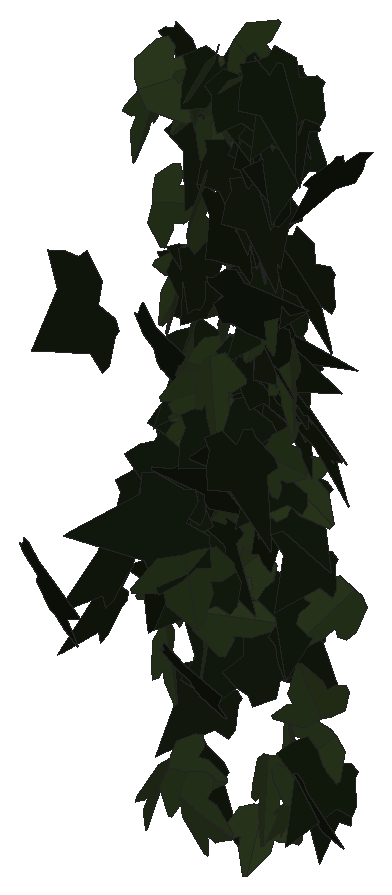
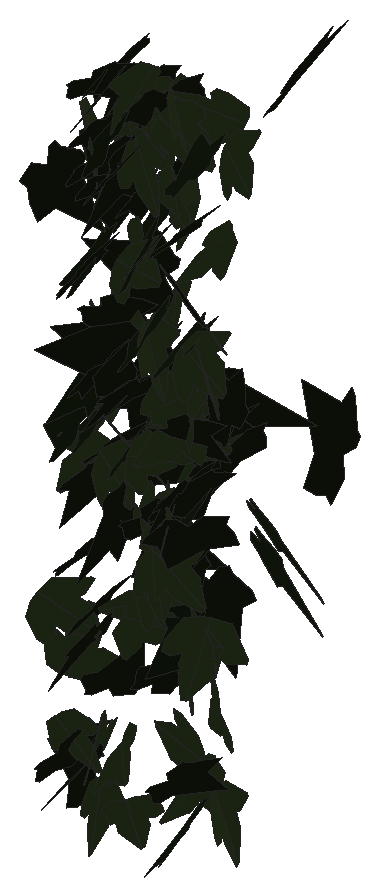
# SketchUp Ruby script. Lengths in inches.
U = 1.inch
M = Sketchup.active_model
def pt(a) = Geom::Point3d.new(a.map { |v| v * U })
def face(e, loops, mat)
  f = e.add_face(loops[0].map { |a| pt(a) })
  loops[1..].each { |l| e.add_face(l.map { |a| pt(a) }).erase! }
  f.material = f.back_material = mat if mat
  f
end
# faces: each face lists its corners as indices into pts; further lists are holes
def faces(e, pts, list, mat = nil) = list.each { |f| face(e, (f[0].is_a?(Array) ? f : [f]).map { |l| l.map { |i| pts[i] } }, mat) }
# xy, xz, yz: faces in a plane at the given z, y or x. An outline is a flat list of corners, or four numbers for a rectangle; further outlines are holes
def ring(l) = l.size == 4 ? [[l[0], l[1]], [l[2], l[1]], [l[2], l[3]], [l[0], l[3]]] : l.each_slice(2).to_a
def flat(e, list, mat, &to3) = list.each { |f| face(e, (f[0].is_a?(Array) ? f : [f]).map { |l| ring(l).map { |u, v| to3.(u, v) } }, mat) }
def xy(e, z, list, mat = nil) = flat(e, list, mat) { |x, y| [x, y, z] }
def xz(e, y, list, mat = nil) = flat(e, list, mat) { |x, z| [x, y, z] }
def yz(e, x, list, mat = nil) = flat(e, list, mat) { |y, z| [x, y, z] }
def lines(e, pts, list) = list.each { |a, b| e.add_line(pt(pts[a]), pt(pts[b])) }
# prism: a flat outline (further loops are holes) pulled along v
def prism(e, loops, v, mat = nil)
  f = face(e, loops, mat); d = Geom::Vector3d.new(v.map { |x| x * U })
  f.pushpull(f.normal.samedirection?(d) ? d.length : -d.length)
end
def box(e, o, s, mat = nil) = prism(e, [[o, [o[0] + s[0], o[1], o[2]], [o[0] + s[0], o[1] + s[1], o[2]], [o[0], o[1] + s[1], o[2]]]], [0, 0, s[2]], mat)
def at(x, y, z, deg = 0) = Geom::Transformation.translation(pt([x, y, z])) * Geom::Transformation.rotation(ORIGIN, Z_AXIS, deg.degrees)
def axes(o, x, y, z) = Geom::Transformation.new([*x, 0, *y, 0, *z, 0, *pt(o).to_a, 1])
def part(name) = M.definitions.add(name)
# library, detail: a bought-in or finely detailed component or shape, given as its bounding box
def library(name, o, s) = part(name).tap { |d| box(d.entities, o, s) }
def detail(e, o, s) = box(e.add_group.entities, o, s)
def put(e, d, t, mat = nil) = e.add_instance(d, t).tap { |i| i.material = mat if mat }
def group(e, t, mat = nil) = e.add_group.tap { |g| g.transformation = t; g.material = mat if mat }.entities
root = M.entities
M.materials.add("efeu1").color = [18, 25, 13]
M.materials.add("efeu2").color = [43, 57, 29]
c1 = part("ivyleaf_9")
p = [[1.54,2.16,1.25],[1.36,2.04,1.19],[-0.21,0.99,0.68],[-0.71,1.11,0.82],[-0.85,0.86,0.67],[-0.8,0.17,0.21],
  [-0.9,-0.01,0.1],[-0.67,-0.16,-0.02],[-0.08,-0.08,-0.05],[-0.03,-0.6,-0.4],[0.65,-0.88,-0.66],[0.83,-0.6,-0.49],
  [1.29,-0.42,-0.43],[1.8125,-0.07,-0.26],[1.21,0.44,0.15]]
faces(c1.entities,p,[[0,1,2,3,4,5,6,7,8,9,10,11,12,13,14]],"efeu1")
c2 = part("ivyleaf_10")
p = [[0,0.5,-0.03],[-0.0625,2.02,-0.43],[-0.19,2.01,-0.46],[-0.54,1.05,-0.29],[-0.52,0.625,-0.18],[-0.83,0.76,-0.28],
  [-1.16,0.64,-0.33],[-1.15,0.33,-0.24],[-0.77,-0.39,0.02],[-0.3,-0.51,0.16],[0.04,-0.48,0.23],[-0.02,2.01,-0.4375],
  [-0.06,2.01,-0.43],[0.04,-0.49,0.23],[0.67,-0.49,0.14],[1.38,0.36,-0.2],[1.375,0.51,-0.24],[0.81,0.65,-0.19],
  [0.62,0.59,-0.15],[0.6,1.09,-0.28],[0.5,1.23,-0.31]]
faces(c2.entities,p,[[0,1,2,3,4,5,6,7,8,9,10],[11,12,0,13,14,15,16,17,18,19,20]],"efeu2")
put(root,c1,axes([526.1875,125.88,202.45],[-0.31024,-0.57511,0.96356],[-0.14685,-0.9703,-0.62642],[1.11249,-0.28846,0.18602]))
put(root,c1,axes([523.3,127.2,192.88],[0.72923,-0.18794,-0.82004],[0.82789,-0.03275,0.74371],[-0.14967,-1.09689,0.1183]))
put(root,c1,axes([526.24,129.36,194.54],[-0.22639,-0.35158,-0.98103],[-0.58216,-0.79,0.41746],[-0.86436,0.62416,-0.02422]))
put(root,c2,axes([526.59,129.14,193.49],[-0.68147,-0.81371,-0.15005],[0.09611,0.11523,-1.06138],[0.82183,-0.68822,-0.0003]))
put(root,c1,axes([523.47,130.27,191.25],[-0.83053,0.51141,-0.15074],[0.12634,-0.0823,-0.97535],[-0.51797,-0.84008,0.00379]))
put(root,c1,axes([523.47,130.41,192.25],[-0.87262,0.45668,-0.06416],[0.05483,-0.03359,-0.98488],[-0.45789,-0.87433,0.00433]))
put(root,c1,axes([524.65,131.27,194.63],[-0.34912,-0.72966,0.43215],[-0.07204,-0.44014,-0.80134],[0.84497,-0.339,0.11024]))
put(root,c1,axes([526.88,130.87,196.27],[0.31389,-0.8535,-0.21236],[-0.05204,0.20706,-0.90912],[0.87798,0.31741,0.02204]))
put(root,c1,axes([524.16,130.8,194.3125],[0.15654,-0.80255,-0.41602],[-0.07249,0.40971,-0.81765],[0.90106,0.17239,0.0065]))
put(root,c2,axes([526.11,130.83,198.21],[-0.04464,0.88501,-0.17145],[0.0101,-0.17115,-0.88614],[-0.90141,-0.04574,-0.00144]))
put(root,c2,axes([524.9375,131.48,184.92],[-0.03387,0.03819,-0.96645],[0.80172,-0.53985,-0.04943],[-0.54105,-0.80233,-0.01274]))
put(root,c1,axes([525.09,131.56,194.05],[0.99147,0.26607,0.22449],[-0.2232,-0.03415,1.02627],[0.26716,-1.016,0.02429]))
put(root,c1,axes([524.48,131.93,188.1875],[0.00264,-0.4091,0.7989],[0.56245,-0.62183,-0.32029],[0.69946,0.50157,0.25453]))
put(root,c1,axes([525.43,132.5,201.48],[-0.20895,-0.43201,0.83597],[0.11627,-0.86162,-0.4162],[0.93379,0.01062,0.23888]))
put(root,c1,axes([525.63,131.89,196.21],[-0.03985,-0.80628,-0.50177],[0.02616,0.50109,-0.80726],[0.9493,-0.04766,0.00118]))
put(root,c1,axes([525.08,132.36,191.51],[-0.55338,-0.49747,0.25851],[-0.19047,-0.17479,-0.74411],[0.52728,-0.58524,0.00251]))
put(root,c2,axes([522.72,132.55,204.46],[0.10439,-0.73708,0.41387],[0.19777,-0.38414,-0.73402],[0.82186,0.18606,0.12406]))
put(root,c1,axes([525.49,132.17,199.68],[0.53828,0.21175,-0.63507],[0.51598,0.38797,0.56669],[0.42652,-0.73657,0.11592]))
put(root,c2,axes([524.6875,132.6,195.76],[0.46548,0.32847,-0.70126],[-0.61611,-0.33857,-0.56755],[-0.46911,0.77059,0.04956]))
put(root,c2,axes([524.88,131.67,201.92],[0.23509,-0.28858,0.96722],[-0.57821,0.77551,0.37192],[-0.82732,-0.62399,0.01491]))
put(root,c1,axes([523.73,132.27,190.89],[0.40174,0.40152,-0.67045],[-0.46155,-0.48643,-0.56788],[-0.63063,0.61179,-0.01149]))
put(root,c2,axes([523.21,132.11,205.25],[0.38958,-0.03538,-0.83311],[0.80143,0.26982,0.36331],[0.23027,-0.87922,0.14501]))
put(root,c1,axes([526.42,132.79,206.14],[0.23417,-0.82718,-0.10521],[-0.0046,0.10799,-0.85933],[0.83383,0.2329,0.02481]))
put(root,c2,axes([522.92,132.75,184.62],[0.22313,-0.83713,0.09685],[0.01325,-0.09669,-0.86627],[0.84261,0.22319,-0.01203]))
put(root,c1,axes([526.48,133.29,194.55],[-0.367,-0.62396,0.42429],[-0.04462,-0.45304,-0.70484],[0.75323,-0.33085,0.16498]))
put(root,c2,axes([527.11,132.08,195.57],[-0.04328,0.48159,0.64392],[-0.16413,0.62599,-0.47921],[-0.78716,-0.157,0.06451]))
put(root,c2,axes([524.36,132.83,205.76],[0.27973,-0.8435,0.02444],[0.00788,-0.02313,-0.88868],[0.84382,0.27984,0.0002]))
put(root,c2,axes([524.45,132.63,196.73],[-0.59025,-0.66652,-0.1353],[0.09503,0.09656,-0.89027],[0.67344,-0.59781,0.00704]))
put(root,c2,axes([525.41,132.82,205.58],[-0.03687,-0.89126,0.02368],[-0.00247,-0.0236,-0.89203],[0.89158,-0.03692,-0.0015]))
put(root,c1,axes([522.39,133.1,196.73],[0.05952,-0.17813,0.8059],[0.45003,-0.67031,-0.1814],[0.69186,0.45133,0.04866]))
put(root,c1,axes([524.3,132.76,192.25],[-0.21052,-0.10092,-0.86869],[0.76003,0.42089,-0.23309],[0.43262,-0.78854,-0.01324]))
put(root,c1,axes([525.93,133.09,202.42],[0.06304,-0.8391,-0.12858],[0,0.12893,-0.84142],[0.8489,0.06231,0.00955]))
put(root,c2,axes([524.94,132.43,190.14],[-0.15686,-0.14478,-0.90391],[0.8091,0.40706,-0.20561],[0.42821,-0.82216,0.05738]))
put(root,c1,axes([525.59,132.7,205.91],[0.15962,-0.61305,-0.58444],[-0.01908,0.59197,-0.62616],[0.84678,0.1289,0.09606]))
put(root,c2,axes([524.22,133.3,205.14],[-0.16822,-0.65469,0.56834],[-0.16508,-0.54416,-0.6757],[0.8511,-0.23494,-0.01873]))
put(root,c2,axes([523.74,132.36,185.13],[0.01643,-0.49016,-0.7341],[0.3509,0.67734,-0.44441],[0.80995,-0.28351,0.20743]))
put(root,c2,axes([526.64,133.15,197.79],[0.62978,-0.31022,0.57392],[0.53127,-0.21911,-0.70141],[0.37864,0.8234,0.02958]))
put(root,c2,axes([524.16,132.8,188.82],[0.5072,-0.51492,-0.27783],[-0.12437,0.2644,-0.71708],[0.57172,0.51432,0.09049]))
put(root,c1,axes([524.95,133.21,203.11],[0.10996,-0.84086,-0.06432],[-0.01117,0.06341,-0.84802],[0.84325,0.11048,-0.00284]))
put(root,c2,axes([523.2,132.37,201.62],[0.12093,-0.37086,-0.76013],[0.31827,0.73137,-0.30619],[0.7836,-0.23983,0.24167]))
put(root,c1,axes([526.68,133.52,205.89],[-0.45853,-0.67369,0.15156],[-0.03732,-0.15748,-0.81295],[0.68952,-0.45653,0.05678]))
put(root,c1,axes([524.35,132.625,199.6],[-0.41181,0.50465,0.61171],[-0.39771,0.46488,-0.65127],[-0.68606,-0.57242,0.01037]))
put(root,c1,axes([524.64,133.07,205.88],[0.03779,-0.81992,-0.44115],[-0.02763,0.44033,-0.82077],[0.93066,0.04636,-0.00645]))
put(root,c2,axes([526.03,133.22,185.44],[-0.05347,0.80361,-0.41174],[0.03399,-0.41038,-0.80536],[-0.90231,-0.06308,-0.00594]))
put(root,c1,axes([526.49,133.43,205.41],[0.22609,-0.81824,0.17506],[0.03522,-0.17187,-0.84882],[0.83601,0.22852,-0.01158]))
put(root,c2,axes([524.76,133.68,193.06],[0.01624,-0.00866,-0.82731],[0.00464,-0.82745,0.00875],[-0.82734,-0.00481,-0.01619]))
put(root,c2,axes([525.98,133.04,205.15],[-0.06327,0.00925,0.89983],[-0.89439,-0.10006,-0.06186],[0.09918,-0.89648,0.01619]))
put(root,c2,axes([525.95,133.11,198.95],[0.69703,-0.3506,-0.20457],[-0.1713,0.11448,-0.77985],[0.368,0.71735,0.02447]))
put(root,c2,axes([524.97,133.23,192.66],[0.83276,-0.33134,-0.01417],[-0.01395,0.00326,-0.89626],[0.33135,0.83288,-0.00213]))
put(root,c2,axes([527.5,133.38,187.75],[-0.55635,-0.51743,-0.29505],[-0.21961,-0.1971,0.75976],[-0.55368,0.5981,-0.00488]))
put(root,c1,axes([523.48,133.79,193.41],[-0.19956,-0.3993,0.67243],[0.05096,-0.69914,-0.40004],[0.78039,-0.05645,0.19808]))
put(root,c2,axes([526.17,133.52,194.28],[0.00977,-0.73463,0.36837],[0.04778,-0.36727,-0.73369],[0.82043,0.03014,0.03834]))
put(root,c1,axes([524.71,133.34,188.05],[-0.43213,-0.66872,0.03372],[0.05848,0.00228,0.79475],[-0.66701,0.43344,0.04784]))
put(root,c2,axes([522.35,133.5,187.93],[0.44406,-0.23107,0.71757],[0.65902,-0.28539,-0.49973],[0.36605,0.79413,0.0292]))
put(root,c2,axes([525.62,133.33,183.88],[0.54261,0.47618,-0.15139],[-0.10529,-0.10951,-0.72182],[-0.48845,0.55259,-0.01259]))
put(root,c2,axes([523.34,133.01,189.5625],[0.35766,-0.04272,0.68291],[-0.65158,0.21396,0.35464],[-0.20887,-0.74061,0.06307]))
put(root,c1,axes([526.13,133.82,202.44],[-0.18224,0.04344,0.83239],[-0.25183,-0.81511,-0.0126],[0.79457,-0.24838,0.18692]))
put(root,c1,axes([526.35,133.29,195.42],[-0.73277,0.39345,0.13631],[-0.13044,0.04512,-0.83144],[-0.39544,-0.74398,0.02166]))
put(root,c1,axes([526.65,133.51,200.4375],[0.47512,-0.70325,0.08184],[0.04447,-0.06873,-0.84871],[0.7066,0.47719,-0.00162]))
put(root,c1,axes([525.98,133.28,197.63],[0.40563,-0.06626,-0.7522],[0.67874,0.40619,0.33024],[0.33092,-0.7519,0.24468]))
put(root,c2,axes([524.41,133.6,195.7],[0.21872,0.23197,-0.72314],[-0.662,-0.31052,-0.29984],[-0.37214,0.68873,0.10837]))
put(root,c2,axes([523.03,133.92,196.99],[-0.0455,0.1218,-0.82294],[0.15439,-0.80861,-0.12822],[-0.81745,-0.1595,0.02159]))
put(root,c1,axes([526.72,133.6,184.91],[0.36377,0.01777,-0.7644],[0.76416,0.02044,0.36414],[0.0261,-0.8463,-0.00726]))
put(root,c1,axes([523.45,134.13,198.7],[-0.25493,-0.59695,0.62262],[0.11902,-0.66737,-0.59113],[0.85431,-0.08516,0.26815]))
put(root,c1,axes([525.17,134.07,195.07],[-0.1813,-0.45814,0.65721],[0.0293,-0.67717,-0.46397],[0.8006,-0.07896,0.1658]))
put(root,c1,axes([526.53,133.36,193.9],[0.13878,-0.65462,-0.50206],[-0.00575,0.50833,-0.6644],[0.82496,0.11367,0.07983]))
put(root,c1,axes([524.59,133.97,193.41],[-0.48584,-0.58124,0.26966],[-0.17409,-0.20594,-0.75755],[0.61665,-0.51608,-0.00141]))
put(root,c1,axes([526.02,133.87,199.27],[-0.64549,-0.4653,0.11034],[-0.09447,-0.05764,-0.79567],[0.46878,-0.65231,-0.0084]))
put(root,c1,axes([526.48,133.39,197.05],[0.79657,-0.43222,-0.08362],[-0.07198,0.04268,-0.90627],[0.43432,0.79981,0.00317]))
put(root,c2,axes([526.71,133.15,194.35],[0.40305,0.48503,0.5669],[0.35681,0.44056,-0.63061],[-0.65522,0.53826,0.00531]))
put(root,c2,axes([525.18,133.58,201.37],[-0.44284,0.63108,-0.3677],[0.21968,-0.29501,-0.7709],[-0.69656,-0.49425,-0.00936]))
put(root,c2,axes([522.99,133.36,190.09],[-0.68465,-0.55594,-0.24115],[0.18401,0.15593,-0.88192],[0.57737,-0.70893,-0.00488]))
put(root,c2,axes([525.79,133.41,204.29],[0.20804,0.08406,0.87164],[-0.87385,-0.03797,0.21223],[0.05659,-0.89532,0.07283]))
put(root,c1,axes([526.72,134.18,200.18],[-0.15773,-0.66543,0.51155],[-0.0264,-0.51631,-0.67977],[0.83892,-0.14137,0.07479]))
put(root,c2,axes([522.76,133.7,198.66],[0.4694,-0.69261,0.04582],[0.02169,-0.04066,-0.83667],[0.69379,0.46988,-0.00485]))
put(root,c2,axes([524.24,133.95,191.25],[-0.0749,-0.68433,0.41502],[0.04414,-0.41973,-0.68413],[0.79912,-0.04096,0.07669]))
put(root,c1,axes([526.06,134.09,203.91],[-0.17396,-0.85389,0.14448],[0.0129,-0.1499,-0.87042],[0.86593,-0.16931,0.04199]))
put(root,c1,axes([523.19,134.05,194.66],[-0.20135,-0.86009,0.05611],[-0.00886,-0.05555,-0.88334],[0.86187,-0.20151,0.00403]))
put(root,c1,axes([523.55,132.95,189.87],[0.30733,0.52797,0.47533],[0.19801,0.43372,-0.60977],[-0.68226,0.3637,0.03714]))
put(root,c1,axes([523.6,134.07,196.48],[-0.67361,-0.47936,0.12079],[-0.09114,-0.08023,-0.82667],[0.48587,-0.67964,0.01239]))
put(root,c1,axes([525.29,133.51,197.02],[0.51327,-0.53082,-0.30203],[-0.10809,0.30934,-0.72736],[0.60109,0.50889,0.1271]))
put(root,c2,axes([522.87,134.09,198.93],[-0.14638,-0.67822,0.52747],[0.02525,-0.53823,-0.68505],[0.85882,-0.09977,0.11005]))
put(root,c1,axes([526.2,134.21,190.1],[-0.02507,-0.75344,0.28147],[0.02492,-0.2822,-0.75317],[0.80391,-0.01475,0.03212]))
put(root,c1,axes([526.63,134.33,191.6875],[-0.25632,-0.63785,0.44543],[-0.02975,-0.46061,-0.67669],[0.77742,-0.22793,0.12097]))
put(root,c2,axes([524.96,134.25,201.06],[-0.17847,-0.46877,0.64152],[0.12514,-0.66588,-0.45176],[0.78462,-0.00043,0.21797]))
put(root,c1,axes([526.83,134.04,195.51],[0.42769,-0.66231,0.33188],[0.18864,-0.27322,-0.78834],[0.71639,0.46735,0.00945]))
put(root,c2,axes([523.93,133.55,202.95],[0.82342,-0.1898,0.24829],[-0.2261,0.12125,0.84253],[-0.21575,-0.85145,0.06463]))
put(root,c1,axes([527.12,134.39,185.5],[-0.28233,-0.77442,0.35747],[-0.12553,-0.33472,-0.82427],[0.84365,-0.30897,-0.00302]))
put(root,c1,axes([523.29,134.36,202.55],[-0.21304,-0.72041,0.36821],[0.05361,-0.39249,-0.7369],[0.80727,-0.16406,0.14611]))
put(root,c1,axes([526.01,133.96,197.5625],[0.17712,-0.79812,-0.13693],[-0.03051,0.13349,-0.81754],[0.80921,0.17973,-0.00085]))
put(root,c1,axes([525.61,134.12,203.59],[-0.16262,-0.80249,-0.07161],[0.01213,0.07061,-0.8188],[0.80558,-0.16306,-0.00212]))
put(root,c2,axes([526.65,133.5,185.11],[-0.2527,0.81695,-0.29826],[-0.10676,0.27911,0.85494],[0.86311,0.27371,0.01843]))
put(root,c2,axes([523.59,134.28,193.77],[-0.04453,0.21512,-0.78538],[0.23813,-0.74873,-0.21858],[-0.77872,-0.24126,-0.02193]))
put(root,c1,axes([525.59,133.625,197.92],[0.63861,-0.13386,0.59867],[0.59444,-0.07843,-0.65164],[0.15153,0.87182,0.03329]))
put(root,c2,axes([525.16,133.32,206.3],[-0.04401,0.73505,0.5135],[-0.05227,0.51114,-0.73616],[-0.89513,-0.06598,0.01774]))
put(root,c2,axes([524.41,133.94,198.89],[0.17023,-0.85781,0.04092],[-0.00136,-0.04198,-0.87449],[0.85879,0.16997,-0.00949]))
put(root,c1,axes([526,134.17,195.99],[0.30072,-0.69775,0.22613],[0.09484,-0.20536,-0.75977],[0.72732,0.31527,0.00557]))
put(root,c1,axes([524.58,134.36,201.27],[0.19611,-0.63258,0.51761],[0.11774,-0.50489,-0.66164],[0.80884,0.22687,-0.02919]))
put(root,c2,axes([523.87,134.09,192.29],[-0.4483,-0.37107,0.57593],[-0.45231,-0.35666,-0.58187],[0.51459,-0.63676,-0.00971]))
put(root,c1,axes([523.1,133.96,184.5],[0.52748,-0.70618,-0.17102],[-0.08067,0.15311,-0.88103],[0.7221,0.53296,0.0265]))
put(root,c1,axes([525.72,134.15,205.24],[0.05214,-0.82511,-0.16531],[0.02023,0.16681,-0.82621],[0.84127,0.04713,0.03011]))
put(root,c1,axes([522.62,134.52,204.74],[-0.1214,-0.57329,0.59413],[0.21571,-0.60168,-0.5365],[0.79694,0.07553,0.23572]))
put(root,c1,axes([525.44,133.36,203.91],[0.2517,-0.11002,-0.85459],[-0.51127,0.69757,-0.24039],[0.69357,0.55415,0.13293]))
put(root,c1,axes([526.78,134.46,184.76],[0.04719,-0.74972,0.31851],[0.09358,-0.31194,-0.74812],[0.80918,0.0798,0.06795]))
put(root,c2,axes([526.23,133.78,184.29],[-0.0246,-0.73808,-0.3261],[0.06591,0.32332,-0.73677],[0.80421,-0.04907,0.05041]))
put(root,c2,axes([523.53,133.51,196.48],[-0.32813,-0.39133,-0.71261],[0.44179,0.55927,-0.51055],[0.68248,-0.55018,-0.01212]))
put(root,c1,axes([525.9,133.32,192.95],[0.12792,0.11396,-0.8894],[-0.63374,0.64706,-0.00824],[0.63434,0.62347,0.17112]))
put(root,c1,axes([525.73,133.97,187.85],[-0.58626,-0.5293,0.18891],[0.13897,0.12797,0.78984],[-0.54455,0.6025,-0.00181]))
put(root,c2,axes([526.59,133.93,204.85],[0.48574,-0.75982,-0.29221],[-0.12964,0.26373,-0.90127],[0.80368,0.50177,0.03123]))
put(root,c1,axes([524.875,133.89,197.33],[0.32111,-0.6126,-0.45195],[0.05592,0.50817,-0.64907],[0.75922,0.22167,0.23896]))
put(root,c1,axes([522.93,134.15,193.72],[-0.28265,-0.70283,-0.44801],[0.152,0.42167,-0.7574],[0.8195,-0.32062,-0.01404]))
put(root,c2,axes([524.46,134.48,190.57],[0.23884,0.37614,-0.75357],[-0.5069,-0.56134,-0.44084],[-0.67261,0.55661,0.06465]))
put(root,c1,axes([523.05,134.04,195.01],[0.31661,-0.66111,-0.34983],[-0.07308,0.35072,-0.72893],[0.74438,0.31562,0.07723]))
put(root,c1,axes([524.05,134.61,201.94],[0.05454,-0.75642,0.35974],[0.05662,-0.35635,-0.75787],[0.83569,0.07351,0.02787]))
put(root,c1,axes([525.16,134.53,204.01],[0.11513,-0.821,0.17555],[0.05448,-0.16952,-0.8285],[0.83779,0.12385,0.02975]))
put(root,c2,axes([524.19,134.69,195.66],[-0.05361,-0.35188,0.74831],[0.15349,-0.74109,-0.33749],[0.81255,0.11677,0.11313]))
put(root,c1,axes([525.41,134.5,204.85],[0.37458,-0.62369,0.43974],[0.22103,-0.38019,-0.72751],[0.73042,0.4349,-0.00536]))
put(root,c2,axes([524.04,134.18,192.23],[-0.15842,-0.79178,0.00963],[-0.0023,-0.00936,-0.80747],[0.79184,-0.15844,-0.00042]))
put(root,c1,axes([523.1,134.69,186.19],[-0.44843,-0.60059,0.32634],[-0.18522,-0.26892,-0.74945],[0.65795,-0.48505,0.01144]))
put(root,c1,axes([526.26,133.98,189.38],[0.40331,-0.54049,-0.43789],[-0.16136,0.41966,-0.66662],[0.67663,0.42224,0.10203]))
put(root,c2,axes([524.79,134.03,204.43],[-0.62369,0.0715,0.54602],[-0.54612,0.02565,-0.62716],[-0.07073,-0.82853,0.02771]))
put(root,c1,axes([527.47,134.4,203.26],[-0.31124,0.48859,-0.5866],[0.12729,-0.59139,-0.56013],[-0.75274,-0.30203,0.14783]))
put(root,c2,axes([527.18,134.73,190.23],[-0.3759,-0.43601,0.68517],[-0.20635,-0.67895,-0.54526],[0.78548,-0.38702,0.18465]))
put(root,c2,axes([527.07,134.21,186.25],[0.54718,0.00407,-0.49725],[-0.4917,0.11483,-0.54012],[0.07425,0.7304,0.08768]))
put(root,c1,axes([524.01,134.64,199.41],[0.27773,-0.72908,0.27717],[0.10764,-0.25558,-0.78013],[0.77252,0.29773,0.00905]))
